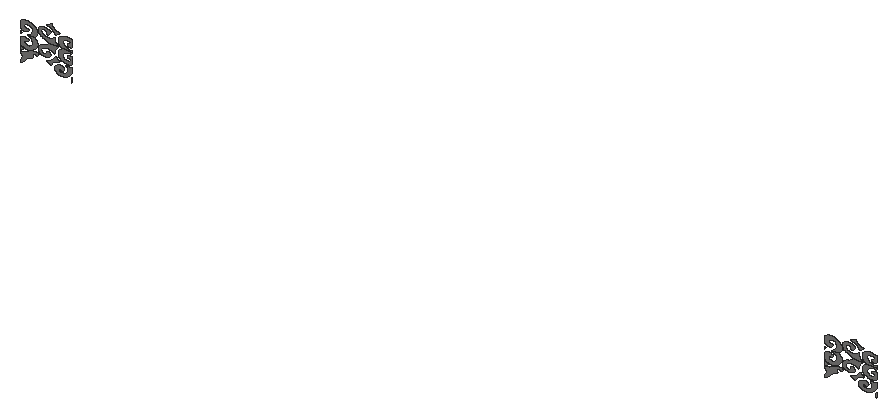
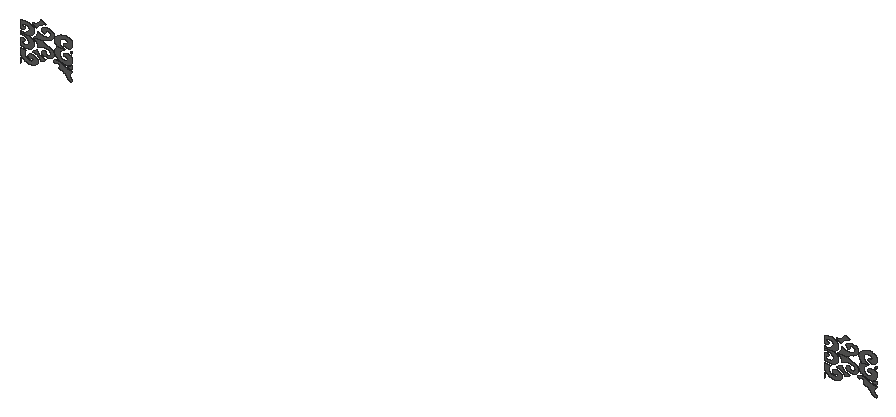
# SketchUp Ruby script. Lengths in inches.
U = 1.inch
M = Sketchup.active_model
def pt(a) = Geom::Point3d.new(a.map { |v| v * U })
def face(e, loops, mat)
  f = e.add_face(loops[0].map { |a| pt(a) })
  loops[1..].each { |l| e.add_face(l.map { |a| pt(a) }).erase! }
  f.material = f.back_material = mat if mat
  f
end
# faces: each face lists its corners as indices into pts; further lists are holes
def faces(e, pts, list, mat = nil) = list.each { |f| face(e, (f[0].is_a?(Array) ? f : [f]).map { |l| l.map { |i| pts[i] } }, mat) }
# xy, xz, yz: faces in a plane at the given z, y or x. An outline is a flat list of corners, or four numbers for a rectangle; further outlines are holes
def ring(l) = l.size == 4 ? [[l[0], l[1]], [l[2], l[1]], [l[2], l[3]], [l[0], l[3]]] : l.each_slice(2).to_a
def flat(e, list, mat, &to3) = list.each { |f| face(e, (f[0].is_a?(Array) ? f : [f]).map { |l| ring(l).map { |u, v| to3.(u, v) } }, mat) }
def xy(e, z, list, mat = nil) = flat(e, list, mat) { |x, y| [x, y, z] }
def xz(e, y, list, mat = nil) = flat(e, list, mat) { |x, z| [x, y, z] }
def yz(e, x, list, mat = nil) = flat(e, list, mat) { |y, z| [x, y, z] }
def lines(e, pts, list) = list.each { |a, b| e.add_line(pt(pts[a]), pt(pts[b])) }
# prism: a flat outline (further loops are holes) pulled along v
def prism(e, loops, v, mat = nil)
  f = face(e, loops, mat); d = Geom::Vector3d.new(v.map { |x| x * U })
  f.pushpull(f.normal.samedirection?(d) ? d.length : -d.length)
end
def box(e, o, s, mat = nil) = prism(e, [[o, [o[0] + s[0], o[1], o[2]], [o[0] + s[0], o[1] + s[1], o[2]], [o[0], o[1] + s[1], o[2]]]], [0, 0, s[2]], mat)
def at(x, y, z, deg = 0) = Geom::Transformation.translation(pt([x, y, z])) * Geom::Transformation.rotation(ORIGIN, Z_AXIS, deg.degrees)
def axes(o, x, y, z) = Geom::Transformation.new([*x, 0, *y, 0, *z, 0, *pt(o).to_a, 1])
def part(name) = M.definitions.add(name)
# library, detail: a bought-in or finely detailed component or shape, given as its bounding box
def library(name, o, s) = part(name).tap { |d| box(d.entities, o, s) }
def detail(e, o, s) = box(e.add_group.entities, o, s)
def put(e, d, t, mat = nil) = e.add_instance(d, t).tap { |i| i.material = mat if mat }
def group(e, t, mat = nil) = e.add_group.tap { |g| g.transformation = t; g.material = mat if mat }.entities
root = M.entities
M.materials.add("[0043_SaddleBrown]4").color = [124, 123, 122]
xz(root,589.17,[[2950.32,580.05,2950.1,580.56,2949.91,581.07,2949.77,581.59,2949.67,582.11,2949.6,582.63,2949.58,583.15,2949.6,583.68,2949.67,584.2,2949.77,584.72,2949.91,585.24,2950.1,585.75,2950.32,586.26],[4200.95,580.05,4200.72,580.56,4200.54,581.07,4200.39,581.59,4200.29,582.11,4200.23,582.63,4200.21,583.15,4200.23,583.68,4200.29,584.2,4200.39,584.72,4200.54,585.24,4200.72,585.75,4200.95,586.26],[2869.93,580.61,2869.93,583.34,2870.95,584.11,2871.81,584.96,2872.49,585.86,2872.98,586.8125,2873.28,587.79,2873.38,588.78,2873.28,589.78,2872.98,590.76,2872.49,591.71,2871.81,592.61,2870.95,593.46,2869.93,594.23,2869.93,595.13,2871.22,595.29,2872.49,595.5,2873.74,595.74,2874.97,596.03,2876.18,596.35,2877.35,596.71,2878.49,597.11,2879.6,597.55,2880.67,598.02,2881.69,598.53,2882.67,599.0625,2883.61,599.63,2884.34,600.07,2885.11,600.47,2885.94,600.83,2886.8,601.16,2887.7,601.46,2888.625,601.71,2889.58,601.92,2890.5625,602.08,2891.56,602.21,2892.57,602.28,2893.58,602.32,2894.6,602.31,2895.41,602.23,2896.17,602.03,2896.85,601.74,2897.4,601.36,2897.79,600.91,2898.01,600.43,2898.05,599.92,2897.9,599.42,2897.57,598.95,2897.08,598.54,2896.46,598.21,2895.73,597.98,2895.62,598.49,2895.3,598.96,2894.79,599.37,2894.125,599.68,2893.35,599.88,2892.52,599.95,2891.7,599.88,2890.92,599.68,2890.26,599.37,2889.75,598.96,2889.43,598.49,2889.32,597.98,2889.28,597.57,2889.25,597.17,2889.24,596.76,2889.25,596.36,2889.28,595.95,2889.32,595.55,2889.39,595.15,2889.47,594.74,2889.5625,594.34,2889.68,593.95,2889.8125,593.55,2889.96,593.15,2888.5,592.79,2887.09,592.36,2885.73,591.86,2884.45,591.3,2883.24,590.67,2882.12,589.99,2881.09,589.26,2880.16,588.48,2879.33,587.65,2878.62,586.79,2878.01,585.89,2877.52,584.97,2877,584.54,2876.45,584.125,2875.89,583.72,2875.3,583.32,2874.69,582.94,2874.06,582.57,2873.42,582.21,2872.76,581.86,2872.07,581.53,2871.375,581.21,2870.66,580.9],[4120.56,580.61,4120.56,583.34,4121.58,584.11,4122.43,584.96,4123.11,585.86,4123.61,586.8125,4123.91,587.79,4124.01,588.78,4123.91,589.78,4123.61,590.76,4123.11,591.71,4122.43,592.61,4121.58,593.46,4120.56,594.23,4120.56,595.13,4121.84,595.29,4123.12,595.5,4124.37,595.74,4125.6,596.03,4126.8,596.35,4127.98,596.71,4129.12,597.11,4130.22,597.55,4131.29,598.02,4132.32,598.53,4133.3,599.0625,4134.23,599.63,4134.96,600.07,4135.74,600.47,4136.56,600.83,4137.42,601.16,4138.32,601.46,4139.25,601.71,4140.21,601.92,4141.1875,602.08,4142.18,602.21,4143.19,602.28,4144.2,602.32,4145.22,602.31,4146.04,602.23,4146.8,602.03,4147.47,601.74,4148.02,601.36,4148.42,600.91,4148.64,600.43,4148.68,599.92,4148.53,599.42,4148.2,598.95,4147.71,598.54,4147.08,598.21,4146.35,597.98,4146.24,598.49,4145.92,598.96,4145.41,599.37,4144.75,599.68,4143.98,599.88,4143.15,599.95,4142.32,599.88,4141.55,599.68,4140.88,599.37,4140.375,598.96,4140.06,598.49,4139.95,597.98,4139.9,597.57,4139.875,597.17,4139.87,596.76,4139.88,596.36,4139.9,595.95,4139.95,595.55,4140.01,595.15,4140.09,594.74,4140.1875,594.34,4140.3,593.95,4140.4375,593.55,4140.59,593.15,4139.125,592.79,4137.71,592.36,4136.36,591.86,4135.08,591.3,4133.87,590.67,4132.75,589.99,4131.72,589.26,4130.79,588.48,4129.96,587.65,4129.24,586.79,4128.64,585.89,4128.15,584.97,4127.625,584.54,4127.08,584.125,4126.51,583.72,4125.92,583.32,4125.32,582.94,4124.69,582.57,4124.04,582.21,4123.38,581.86,4122.7,581.53,4122,581.21,4121.29,580.9],[2933.97,583.36,2932.56,583.46,2931.17,583.66,2929.83,583.96,2927.89,584.61,2926.2,585.48,2924.8125,586.54,2923.78,587.74,2923.15,589.04,2922.93,590.39,2923.15,591.74,2923.78,593.04,2924.8125,594.24,2926.2,595.29,2927.89,596.16,2929.83,596.82,2930.47,597.05,2931.16,597.21,2931.89,597.31,2932.63,597.33,2933.37,597.28,2934.09,597.17,2934.77,596.98,2935.39,596.73,2935.93,596.42,2936.4,596.0625,2936.76,595.66,2937.02,595.23,2937.38,594.85,2937.66,594.45,2937.83,594.02,2937.91,593.58,2937.88,593.14,2937.76,592.7,2937.54,592.28,2937.22,591.89,2936.8125,591.52,2936.33,591.2,2935.77,590.92,2935.16,590.6875,2934.8,590.8,2934.46,590.93,2934.13,591.07,2933.82,591.23,2933.53,591.4,2933.26,591.58,2933.01,591.78,2932.79,591.98,2932.58,592.19,2932.4,592.41,2932.25,592.64,2932.12,592.87,2931.35,592.59,2930.6875,592.22,2930.14,591.79,2929.74,591.3,2929.49,590.77,2929.41,590.23,2929.49,589.68,2929.74,589.15,2930.14,588.66,2930.6875,588.23,2931.35,587.86,2932.12,587.58,2933.05,587.56,2933.98,587.58,2934.91,587.64,2935.83,587.75,2936.73,587.9,2937.61,588.09,2938.47,588.32,2939.29,588.58,2940.09,588.89,2940.84,589.23,2941.55,589.6,2942.21,590,2942.79,590.79,2943.26,591.6,2943.61,592.43,2943.83,593.28,2943.93,594.14,2943.9,595,2943.75,595.85,2943.47,596.7,2943.07,597.52,2942.55,598.32,2941.92,599.09,2941.17,599.82,2941.93,599.65,2942.72,599.53,2943.51,599.46,2944.32,599.42,2945.12,599.43,2945.92,599.48,2946.72,599.57,2947.49,599.7,2948.25,599.88,2948.97,600.09,2949.67,600.35,2950.32,600.64,2950.32,593.03,2949.96,592.48,2949.58,591.93,2949.18,591.39,2948.77,590.85,2948.35,590.3125,2947.9,589.78,2947.45,589.26,2946.97,588.74,2946.49,588.23,2945.99,587.72,2945.47,587.21,2944.94,586.71,2944.08,586.02,2943.1,585.38,2942,584.82,2940.8125,584.34,2939.54,583.95,2938.2,583.66,2936.81,583.46,2935.39,583.36],
  [4184.6,583.36,4183.18,583.46,4181.79,583.66,4180.45,583.96,4178.52,584.61,4176.83,585.48,4175.4375,586.54,4174.41,587.74,4173.77,589.04,4173.56,590.39,4173.77,591.74,4174.41,593.04,4175.4375,594.24,4176.83,595.29,4178.52,596.16,4180.45,596.82,4181.1,597.05,4181.79,597.21,4182.51,597.31,4183.26,597.33,4184,597.28,4184.71,597.17,4185.39,596.98,4186.01,596.73,4186.56,596.42,4187.02,596.0625,4187.39,595.66,4187.64,595.23,4188.01,594.85,4188.28,594.45,4188.46,594.02,4188.53,593.58,4188.51,593.14,4188.38,592.7,4188.16,592.28,4187.84,591.89,4187.4375,591.52,4186.95,591.2,4186.4,590.92,4185.78,590.6875,4185.43,590.8,4185.09,590.93,4184.76,591.07,4184.45,591.23,4184.16,591.4,4183.89,591.58,4183.64,591.78,4183.41,591.98,4183.21,592.19,4183.03,592.41,4182.87,592.64,4182.74,592.87,4181.98,592.59,4181.3125,592.22,4180.77,591.79,4180.36,591.3,4180.12,590.77,4180.03,590.23,4180.12,589.68,4180.36,589.15,4180.77,588.66,4181.3125,588.23,4181.98,587.86,4182.74,587.58,4183.68,587.56,4184.61,587.58,4185.54,587.64,4186.45,587.75,4187.36,587.9,4188.24,588.09,4189.09,588.32,4189.92,588.58,4190.71,588.89,4191.46,589.23,4192.17,589.6,4192.83,590,4193.42,590.79,4193.89,591.6,4194.23,592.43,4194.46,593.28,4194.56,594.14,4194.53,595,4194.375,595.85,4194.1,596.7,4193.69,597.52,4193.17,598.32,4192.54,599.09,4191.8,599.82,4192.56,599.65,4193.34,599.53,4194.14,599.46,4194.94,599.42,4195.75,599.43,4196.55,599.48,4197.34,599.57,4198.12,599.7,4198.87,599.88,4199.6,600.09,4200.29,600.35,4200.95,600.64,4200.95,593.03,4200.58,592.48,4200.2,591.93,4199.81,591.39,4199.4,590.85,4198.97,590.3125,4198.53,589.78,4198.07,589.26,4197.6,588.74,4197.11,588.23,4196.61,587.72,4196.1,587.21,4195.57,586.71,4194.71,586.02,4193.73,585.38,4192.63,584.82,4191.4375,584.34,4190.16,583.95,4188.82,583.66,4187.43,583.46,4186.02,583.36],[2918.45,593.19,2917.9,593.51,2917.34,593.83,2916.78,594.14,2916.2,594.45,2915.61,594.75,2915.02,595.04,2914.42,595.32,2913.81,595.6,2913.1875,595.875,2912.5625,596.14,2911.93,596.4,2911.29,596.65,2912.89,597.11,2914.43,597.64,2915.9,598.25,2917.28,598.92,2918.57,599.66,2919.77,600.46,2920.86,601.32,2921.83,602.23,2922.6875,603.18,2923.42,604.17,2924.02,605.1875,2924.49,606.23,2925.02,605.83,2925.5625,605.43,2926.11,605.04,2926.67,604.66,2927.83,603.9,2928.42,603.53,2929.02,603.17,2929.63,602.8125,2930.25,602.46,2930.88,602.12,2931.52,601.78,2929.85,601.54,2928.24,601.2,2926.69,600.75,2925.23,600.2,2923.88,599.56,2922.64,598.83,2921.55,598.02,2920.59,597.15,2919.8,596.22,2919.17,595.24,2918.72,594.23],[4169.08,593.19,4168.53,593.51,4167.97,593.83,4167.4,594.14,4166.82,594.45,4166.24,594.75,4165.65,595.04,4164.43,595.6,4163.8125,595.875,4163.1875,596.14,4162.55,596.4,4161.91,596.65,4163.51,597.11,4165.05,597.64,4166.52,598.25,4167.91,598.92,4169.2,599.66,4170.39,600.46,4171.48,601.32,4172.46,602.23,4173.3125,603.18,4174.04,604.17,4174.65,605.1875,4175.12,606.23,4175.65,605.83,4176.1875,605.43,4176.74,605.04,4177.3,604.66,4177.87,604.28,4178.45,603.9,4179.04,603.53,4179.65,603.17,4180.26,602.8125,4180.875,602.46,4181.5,602.12,4182.14,601.78,4180.48,601.54,4178.86,601.2,4177.32,600.75,4175.86,600.2,4174.5,599.56,4173.27,598.83,4172.17,598.02,4171.22,597.15,4170.43,596.22,4169.8,595.24,4169.35,594.23],[2869.93,598.4,2869.93,602.86,2870.29,602.55,2870.68,602.26,2871.09,601.99,2871.54,601.73,2872.02,601.49,2872.52,601.28,2873.04,601.08,2873.59,600.91,2874.15,600.76,2874.73,600.64,2875.32,600.54,2875.92,600.46,2875.55,600.18,2875.15,599.91,2874.72,599.66,2874.27,599.43,2873.79,599.22,2873.28,599.03,2872.76,598.87,2872.22,598.73,2871.66,598.61,2871.1,598.51,2870.52,598.45],[4120.56,598.4,4120.56,602.86,4120.91,602.55,4121.3,602.26,4121.72,601.99,4122.17,601.73,4122.64,601.49,4123.15,601.28,4123.67,601.08,4124.21,600.91,4124.77,600.76,4125.35,600.64,4125.94,600.54,4126.54,600.46,4126.17,600.18,4125.78,599.91,4125.35,599.66,4124.89,599.43,4124.41,599.22,4123.91,599.03,4123.39,598.87,4122.85,598.73,4122.29,598.61,4121.72,598.51,4121.14,598.45],
  [2907.9,601.54,2905.91,601.66,2904,602.02,2902.25,602.62,2900.73,603.42,2899.5,604.39,2898.63,605.5,2898.14,606.69,2897.99,607.57,2897.97,608.46,2898.07,609.34,2898.3,610.21,2898.65,611.07,2899.13,611.9,2899.72,612.71,2900.42,613.48,2901.23,614.21,2902.14,614.9,2903.15,615.53,2904.24,616.11,2905.39,616.38,2906.52,616.6875,2907.61,617.04,2908.67,617.42,2909.7,617.84,2910.6875,618.3,2911.63,618.79,2912.53,619.31,2913.375,619.86,2914.17,620.4375,2914.91,621.04,2915.6,621.67,2929.37,621.67,2928.39,620.92,2927.48,620.13,2926.66,619.3,2925.92,618.45,2925.27,617.57,2924.7,616.67,2924.23,615.75,2923.85,614.8125,2923.57,613.86,2923.38,612.9,2923.29,611.9375,2923.3,610.97,2922.72,611.43,2922.08,611.87,2921.4,612.28,2920.68,612.66,2919.91,613,2919.1,613.3125,2918.26,613.59,2917.39,613.83,2916.5,614.03,2915.58,614.1875,2914.65,614.31,2913.71,614.39,2912.08,614.41,2910.47,614.28,2908.91,613.99,2907.45,613.55,2906.12,612.98,2904.94,612.29,2903.96,611.49,2903.2,610.61,2902.67,609.66,2902.39,608.68,2902.37,607.68,2902.6,606.69,2902.85,606.21,2903.25,605.76,2903.77,605.36,2904.4,605.02,2905.11,604.76,2905.89,604.59,2906.71,604.5,2907.54,604.51,2908.36,604.61,2909.13,604.8,2909.84,605.07,2910.45,605.41,2910.61,605.62,2910.76,605.83,2910.88,606.05,2910.98,606.27,2911.07,606.5,2911.13,606.73,2911.17,606.96,2911.19,607.1875,2911.2,607.42,2911.18,607.65,2911.14,607.88,2911.08,608.11,2911.04,608.32,2911.07,608.53,2911.15,608.74,2911.29,608.93,2911.48,609.11,2911.72,609.26,2912,609.39,2912.31,609.48,2912.64,609.54,2912.98,609.56,2913.33,609.55,2913.67,609.5,2914.27,609.21,2914.82,608.88,2915.3125,608.51,2915.73,608.11,2916.08,607.69,2916.35,607.25,2916.54,606.79,2916.65,606.32,2916.67,605.84,2916.61,605.37,2916.47,604.91,2916.25,604.45,2915.04,603.47,2913.54,602.66,2911.8,602.05,2909.89,601.67],[4158.53,601.54,4156.53,601.66,4154.62,602.02,4152.87,602.62,4151.35,603.42,4150.13,604.39,4149.25,605.5,4148.76,606.69,4148.61,607.57,4148.59,608.46,4148.7,609.34,4148.93,610.21,4149.28,611.07,4149.75,611.9,4150.34,612.71,4151.05,613.48,4151.86,614.21,4152.77,614.9,4153.77,615.53,4154.86,616.11,4156.02,616.38,4157.14,616.6875,4158.24,617.04,4159.3,617.42,4160.33,617.84,4161.3125,618.3,4162.25,618.79,4163.15,619.31,4164,619.86,4164.8,620.4375,4165.54,621.04,4166.22,621.67,4179.99,621.67,4179.01,620.92,4178.11,620.13,4177.28,619.3,4176.54,618.45,4175.89,617.57,4175.33,616.67,4174.86,615.75,4174.48,614.8125,4174.2,613.86,4174.01,612.9,4173.92,611.9375,4173.92,610.97,4173.34,611.43,4172.71,611.87,4172.03,612.28,4171.3,612.66,4170.53,613,4169.73,613.3125,4168.89,613.59,4168.02,613.83,4167.125,614.03,4166.21,614.1875,4165.28,614.31,4164.33,614.39,4162.71,614.41,4161.1,614.28,4159.54,613.99,4158.08,613.55,4156.74,612.98,4155.57,612.29,4154.59,611.49,4153.83,610.61,4153.3,609.66,4153.02,608.68,4152.99,607.68,4153.22,606.69,4153.48,606.21,4153.87,605.76,4154.39,605.36,4155.02,605.02,4155.74,604.76,4156.52,604.59,4157.34,604.5,4158.17,604.51,4158.98,604.61,4159.76,604.8,4160.46,605.07,4161.08,605.41,4161.24,605.62,4161.38,605.83,4161.5,606.05,4161.61,606.27,4161.69,606.5,4161.75,606.73,4161.8,606.96,4161.82,607.1875,4161.82,607.42,4161.8,607.65,4161.76,607.88,4161.7,608.11,4161.67,608.32,4161.69,608.53,4161.77,608.74,4161.91,608.93,4162.11,609.11,4162.35,609.26,4162.625,609.39,4162.93,609.48,4163.27,609.54,4163.61,609.56,4163.95,609.55,4164.29,609.5,4164.9,609.21,4165.45,608.88,4165.9375,608.51,4166.36,608.11,4166.7,607.69,4166.97,607.25,4167.16,606.79,4167.27,606.32,4167.3,605.84,4167.24,605.37,4167.09,604.91,4166.87,604.45,4165.67,603.47,4164.16,602.66,4162.42,602.05,4160.52,601.67],[2880.76,601.96,2879.19,601.97,2877.65,602.14,2876.16,602.44,2874.77,602.89,2873.5,603.45,2872.38,604.13,2871.45,604.91,2870.72,605.76,2870.21,606.67,2869.93,607.62,2869.93,614.39,2870.39,615.13,2871.07,615.8,2871.95,616.38,2872.98,616.85,2874.14,617.19,2875.38,617.38,2876.67,617.44,2877.94,617.34,2879.16,617.09,2880.29,616.71,2881.28,616.21,2882.09,615.6,2882.33,615.33,2882.49,615.03,2882.56,614.73,2882.54,614.42,2882.43,614.11,2882.23,613.83,2881.95,613.57,2881.59,613.35,2881.18,613.17,2880.73,613.04,2880.24,612.96,2879.74,612.9375,2879.07,612.91,2878.42,612.8125,2877.8125,612.65,2877.26,612.42,2876.78,612.14,2876.38,611.81,2876.08,611.44,2875.89,611.05,2875.81,610.64,2875.85,610.23,2876.01,609.83,2876.27,609.45,2876.65,608.8,2877.22,608.21,2877.97,607.6875,2878.86,607.26,2879.87,606.95,2880.95,606.75,2882.07,606.69,2883.2,606.76,2884.28,606.95,2885.28,607.27,2886.7,608.37,2887.84,609.6,2888.65,610.92,2889.12,612.3,2889.25,613.7,2889.02,615.1,2888.45,616.47,2887.54,617.76,2886.32,618.96,2884.82,620.02,2883.07,620.9375,2881.12,621.67,2892.0625,621.67,2893.89,620.09,2895.29,618.34,2896.22,616.49,2896.66,614.57,2896.6,612.625,2896.04,610.71,2895,608.88,2893.5,607.17,2891.58,605.625,2889.29,604.29,2886.68,603.1875,2883.82,602.36,2882.32,602.08],[4131.39,601.96,4129.82,601.97,4128.27,602.14,4126.79,602.44,4125.39,602.89,4124.12,603.45,4123.01,604.13,4122.08,604.91,4121.35,605.76,4120.84,606.67,4120.56,607.62,4120.56,614.39,4121.02,615.13,4121.7,615.8,4122.57,616.38,4123.61,616.85,4124.77,617.19,4126.01,617.38,4127.29,617.44,4128.57,617.34,4129.79,617.09,4130.91,616.71,4131.9,616.21,4132.72,615.6,4132.96,615.33,4133.12,615.03,4133.18,614.73,4133.16,614.42,4133.05,614.11,4132.85,613.83,4132.57,613.57,4132.22,613.35,4131.81,613.17,4131.35,613.04,4130.86,612.96,4130.36,612.9375,4129.7,612.91,4129.05,612.8125,4128.4375,612.65,4127.88,612.42,4127.4,612.14,4127,611.81,4126.71,611.44,4126.52,611.05,4126.44,610.64,4126.48,610.23,4126.63,609.83,4126.89,609.45,4127.27,608.8,4127.85,608.21,4128.59,607.6875,4129.48,607.26,4130.49,606.95,4131.57,606.75,4132.7,606.69,4133.82,606.76,4134.9,606.95,4135.91,607.27,4137.33,608.37,4138.46,609.6,4139.27,610.92,4139.75,612.3,4139.87,613.7,4139.64,615.1,4139.07,616.47,4138.17,617.76,4136.95,618.96,4135.45,620.02,4133.7,620.9375,4131.74,621.67,4142.6875,621.67,4144.52,620.09,4145.91,618.34,4146.84,616.49,4147.28,614.57,4147.23,612.625,4146.67,610.71,4145.63,608.88,4144.13,607.17,4142.21,605.625,4139.91,604.29,4137.31,603.1875,4134.45,602.36,4132.94,602.08],[2942.6,603.16,2939.9,603.34,2937.31,603.85,2934.93,604.66,2932.86,605.74,2931.17,607.05,2929.94,608.54,2929.21,610.15,2929.02,611.82,2929.35,613.47,2929.43,614.32,2929.64,615.16,2929.97,615.98,2930.42,616.78,2930.98,617.56,2931.66,618.3,2932.45,618.99,2933.34,619.64,2934.32,620.24,2935.38,620.78,2936.52,621.26,2937.73,621.67,2950.32,621.67,2950.32,619.15,2950.02,619.38,2949.68,619.6,2949.3,619.78,2948.88,619.9375,2948.4375,620.0625,2947.98,620.15,2947.5,620.21,2947.01,620.23,2946.53,620.22,2946.05,620.17,2945.58,620.09,2945.13,619.97,2944.05,619.61,2943.02,619.2,2942.03,618.75,2941.1,618.26,2940.24,617.73,2939.43,617.15,2938.7,616.55,2938.04,615.91,2937.45,615.25,2936.95,614.5625,2936.52,613.85,2936.1875,613.13,2935.99,612.42,2935.96,611.71,2936.1,610.99,2936.4,610.3,2936.87,609.64,2937.48,609.04,2938.24,608.49,2939.11,608.01,2940.09,607.62,2941.15,607.32,2942.27,607.11,2943.42,607.01,2944.49,607.04,2945.5,607.24,2946.41,607.58,2947.16,608.04,2947.7,608.61,2948,609.23,2948.04,609.89,2947.82,610.53,2947.35,611.12,2946.66,611.62,2945.8,612,2944.8,612.24,2944.56,612.22,2944.3125,612.24,2944.07,612.27,2943.85,612.34,2943.65,612.42,2943.47,612.53,2943.33,612.65,2943.22,612.79,2943.15,612.93,2943.125,613.08,2943.14,613.24,2943.2,613.38,2943.48,613.79,2943.875,614.17,2944.36,614.5,2944.92,614.78,2945.56,615,2946.24,615.15,2946.95,615.23,2947.68,615.24,2948.4,615.18,2949.09,615.05,2949.74,614.85,2950.32,614.58,2950.32,604.55,2947.92,603.77,2945.31,603.3],
  [4193.22,603.16,4190.52,603.34,4187.93,603.85,4185.55,604.66,4183.48,605.74,4181.8,607.05,4180.57,608.54,4179.84,610.15,4179.64,611.82,4179.98,613.47,4180.06,614.32,4180.26,615.16,4180.59,615.98,4181.04,616.78,4181.61,617.56,4182.29,618.3,4183.08,618.99,4183.96,619.64,4184.94,620.24,4186.01,620.78,4187.15,621.26,4188.36,621.67,4200.95,621.67,4200.95,619.15,4200.65,619.38,4200.3,619.6,4199.92,619.78,4199.51,619.9375,4199.0625,620.0625,4198.6,620.15,4198.125,620.21,4197.64,620.23,4197.15,620.22,4196.67,620.17,4196.2,620.09,4195.76,619.97,4194.68,619.61,4193.64,619.2,4192.66,618.75,4191.73,618.26,4190.86,617.73,4190.06,617.15,4189.32,616.55,4188.66,615.91,4188.08,615.25,4187.57,614.5625,4187.15,613.85,4186.8125,613.13,4186.61,612.42,4186.58,611.71,4186.72,610.99,4187.03,610.3,4187.49,609.64,4188.11,609.04,4188.86,608.49,4189.74,608.01,4190.71,607.62,4191.77,607.32,4192.89,607.11,4194.05,607.01,4195.11,607.04,4196.13,607.24,4197.04,607.58,4197.79,608.04,4198.33,608.61,4198.625,609.23,4198.67,609.89,4198.45,610.53,4197.98,611.12,4197.29,611.62,4196.42,612,4195.43,612.24,4195.18,612.22,4194.9375,612.24,4194.7,612.27,4194.47,612.34,4194.27,612.42,4194.1,612.53,4193.95,612.65,4193.84,612.79,4193.78,612.93,4193.75,613.08,4193.77,613.24,4193.82,613.38,4194.11,613.79,4194.5,614.17,4194.98,614.5,4195.55,614.78,4196.18,615,4196.86,615.15,4197.58,615.23,4198.3,615.24,4199.02,615.18,4199.71,615.05,4200.36,614.85,4200.95,614.58,4200.95,604.55,4198.54,603.77,4195.93,603.3],[2869.93,620.2,2869.93,621.67,2872.33,621.67,2872.02,621.66,2871.71,621.62,2871.41,621.5625,2871.13,621.48,2870.87,621.37,2870.63,621.24,2870.43,621.1,2870.25,620.9375,2870.12,620.76,2870.01,620.58,2869.95,620.39],[4120.56,620.2,4120.56,621.67,4122.96,621.67,4122.64,621.66,4122.33,621.62,4122.04,621.5625,4121.76,621.48,4121.5,621.37,4121.26,621.24,4121.05,621.1,4120.88,620.9375,4120.74,620.76,4120.64,620.58,4120.58,620.39],[2869.93,621.67,2872.33,621.67,2872.02,621.6875,2871.71,621.72,2871.41,621.79,2871.13,621.87,2870.87,621.98,2870.63,622.1,2870.43,622.25,2870.25,622.41,2870.12,622.58,2870.01,622.76,2869.95,622.95,2869.93,623.15],[2881.12,621.67,2892.0625,621.67,2893.89,623.26,2895.29,625,2896.22,626.86,2896.66,628.78,2896.6,630.72,2896.04,632.63,2895,634.47,2893.5,636.18,2891.58,637.72,2889.29,639.06,2886.68,640.16,2883.82,640.99,2882.32,641.26,2880.76,641.39,2879.19,641.37,2877.65,641.21,2876.16,640.9,2874.77,640.46,2873.5,639.89,2872.38,639.21,2871.45,638.4375,2870.72,637.59,2870.21,636.67,2869.93,635.73,2869.93,628.95,2870.39,628.22,2871.07,627.55,2871.95,626.97,2872.98,626.5,2874.14,626.16,2875.38,625.96,2876.67,625.91,2877.94,626.01,2879.16,626.25,2880.29,626.63,2881.28,627.14,2882.09,627.75,2882.33,628.02,2882.49,628.3125,2882.56,628.62,2882.54,628.93,2882.43,629.23,2882.23,629.52,2881.95,629.77,2881.59,630,2881.18,630.17,2880.73,630.31,2880.24,630.38,2879.74,630.41,2879.07,630.44,2878.42,630.53,2877.8125,630.7,2877.26,630.93,2876.78,631.21,2876.38,631.54,2876.08,631.91,2875.89,632.3,2875.81,632.71,2875.85,633.12,2876.01,633.51,2876.27,633.89,2876.65,634.54,2877.22,635.14,2877.97,635.66,2878.86,636.08,2879.87,636.4,2880.95,636.59,2882.07,636.66,2883.2,636.59,2884.28,636.4,2885.28,636.08,2886.7,634.97,2887.84,633.75,2888.65,632.43,2889.12,631.05,2889.25,629.64,2889.02,628.24,2888.45,626.875,2887.54,625.58,2886.32,624.39,2884.82,623.32,2883.07,622.41],
  [2915.6,621.67,2929.37,621.67,2928.39,622.43,2927.48,623.22,2926.66,624.04,2925.92,624.89,2925.27,625.77,2924.7,626.68,2924.23,627.6,2923.85,628.53,2923.57,629.48,2923.38,630.44,2923.29,631.41,2923.3,632.375,2922.72,631.91,2922.08,631.47,2921.4,631.07,2920.68,630.6875,2919.91,630.34,2919.1,630.03,2918.26,629.76,2917.39,629.52,2916.5,629.32,2915.58,629.16,2914.65,629.04,2913.71,628.96,2912.08,628.9375,2910.47,629.07,2908.91,629.36,2907.45,629.79,2906.12,630.37,2904.94,631.06,2903.96,631.86,2903.2,632.74,2902.67,633.68,2902.39,634.67,2902.37,635.67,2902.6,636.65,2902.85,637.14,2903.25,637.59,2903.77,637.99,2904.4,638.32,2905.11,638.58,2905.89,638.76,2906.71,638.84,2907.54,638.84,2908.36,638.74,2909.13,638.55,2909.84,638.28,2910.45,637.9375,2910.61,637.73,2910.76,637.51,2910.88,637.29,2910.98,637.07,2911.07,636.85,2911.13,636.62,2911.17,636.39,2911.19,636.16,2911.2,635.93,2911.18,635.7,2911.14,635.47,2911.08,635.24,2911.04,635.03,2911.07,634.82,2911.15,634.61,2911.29,634.42,2911.48,634.24,2911.72,634.09,2912,633.96,2912.31,633.87,2912.64,633.81,2912.98,633.78,2913.33,633.79,2913.67,633.84,2914.27,634.14,2914.82,634.47,2915.3125,634.84,2915.73,635.23,2916.08,635.66,2916.35,636.1,2916.54,636.56,2916.65,637.03,2916.67,637.5,2916.61,637.97,2916.47,638.44,2916.25,638.89,2915.04,639.875,2913.54,640.6875,2911.8,641.29,2909.89,641.67,2907.9,641.8,2905.91,641.6875,2904,641.32,2902.25,640.73,2900.73,639.93,2899.5,638.95,2898.63,637.85,2898.14,636.65,2897.99,635.77,2897.97,634.89,2898.07,634.01,2898.3,633.14,2898.65,632.28,2899.13,631.44,2899.72,630.64,2900.42,629.86,2901.23,629.13,2902.14,628.45,2903.15,627.81,2904.24,627.24,2905.39,626.97,2906.52,626.66,2907.61,626.31,2908.67,625.92,2909.7,625.5,2910.6875,625.05,2911.63,624.56,2912.53,624.04,2913.375,623.49,2914.17,622.91,2914.91,622.3],[2937.73,621.67,2950.32,621.67,2950.32,624.2,2950.02,623.96,2949.68,623.75,2949.3,623.56,2948.88,623.41,2948.4375,623.28,2947.98,623.19,2947.5,623.14,2947.01,623.11,2946.53,623.125,2946.05,623.18,2945.58,623.26,2945.13,623.375,2944.05,623.74,2943.02,624.14,2942.03,624.59,2941.1,625.09,2940.24,625.62,2939.43,626.19,2938.7,626.8,2938.04,627.43,2937.45,628.1,2936.95,628.78,2936.52,629.49,2936.1875,630.22,2935.99,630.92,2935.96,631.64,2936.1,632.35,2936.4,633.04,2936.87,633.7,2937.48,634.3125,2938.24,634.86,2939.11,635.33,2940.09,635.73,2941.15,636.03,2942.27,636.23,2943.42,636.34,2944.49,636.3,2945.5,636.11,2946.41,635.77,2947.16,635.3,2947.7,634.74,2948,634.11,2948.04,633.46,2947.82,632.82,2947.35,632.23,2946.66,631.73,2945.8,631.35,2944.8,631.11,2944.56,631.125,2944.3125,631.11,2944.07,631.07,2943.85,631.01,2943.65,630.92,2943.47,630.82,2943.33,630.69,2943.22,630.56,2943.15,630.41,2943.125,630.26,2943.14,630.11,2943.2,629.96,2943.48,629.55,2943.875,629.18,2944.36,628.85,2944.92,628.57,2945.56,628.35,2946.24,628.2,2946.95,628.11,2947.68,628.1,2948.4,628.16,2949.09,628.3,2949.74,628.5,2950.32,628.76,2950.32,638.8,2947.92,639.57,2945.31,640.04,2942.6,640.1875,2939.9,640,2937.31,639.5,2934.93,638.6875,2932.86,637.61,2931.17,636.29,2929.94,634.8,2929.21,633.2,2929.02,631.53,2929.35,629.875,2929.43,629.03,2929.64,628.1875,2929.97,627.36,2930.42,626.5625,2930.98,625.79,2931.66,625.05,2932.45,624.35,2933.34,623.7,2934.32,623.1,2935.38,622.5625,2936.52,622.09],[4120.56,621.67,4122.96,621.67,4122.64,621.6875,4122.33,621.72,4122.04,621.79,4121.76,621.87,4121.5,621.98,4121.26,622.1,4121.05,622.25,4120.88,622.41,4120.74,622.58,4120.64,622.76,4120.58,622.95,4120.56,623.15],[4131.74,621.67,4142.6875,621.67,4144.52,623.26,4145.91,625,4146.84,626.86,4147.28,628.78,4147.23,630.72,4146.67,632.63,4145.63,634.47,4144.13,636.18,4142.21,637.72,4139.91,639.06,4137.31,640.16,4134.45,640.99,4132.94,641.26,4131.39,641.39,4129.82,641.37,4128.27,641.21,4126.79,640.9,4125.39,640.46,4124.12,639.89,4123.01,639.21,4122.08,638.4375,4121.35,637.59,4120.84,636.67,4120.56,635.73,4120.56,628.95,4121.02,628.22,4121.7,627.55,4122.57,626.97,4123.61,626.5,4124.77,626.16,4126.01,625.96,4127.29,625.91,4128.57,626.01,4129.79,626.25,4130.91,626.63,4131.9,627.14,4132.72,627.75,4132.96,628.02,4133.12,628.3125,4133.18,628.62,4133.16,628.93,4133.05,629.23,4132.85,629.52,4132.57,629.77,4132.22,630,4131.81,630.17,4131.35,630.31,4130.86,630.38,4130.36,630.41,4129.7,630.44,4129.05,630.53,4128.4375,630.7,4127.88,630.93,4127.4,631.21,4127,631.54,4126.71,631.91,4126.52,632.3,4126.44,632.71,4126.48,633.12,4126.63,633.51,4126.89,633.89,4127.27,634.54,4127.85,635.14,4128.59,635.66,4129.48,636.08,4130.49,636.4,4131.57,636.59,4132.7,636.66,4133.82,636.59,4134.9,636.4,4135.91,636.08,4137.33,634.97,4138.46,633.75,4139.27,632.43,4139.75,631.05,4139.87,629.64,4139.64,628.24,4139.07,626.875,4138.17,625.58,4136.95,624.39,4135.45,623.32,4133.7,622.41],[4166.22,621.67,4179.99,621.67,4179.01,622.43,4178.11,623.22,4177.28,624.04,4176.54,624.89,4175.89,625.77,4175.33,626.68,4174.86,627.6,4174.48,628.53,4174.2,629.48,4174.01,630.44,4173.92,631.41,4173.92,632.375,4173.34,631.91,4172.71,631.47,4172.03,631.07,4171.3,630.6875,4170.53,630.34,4169.73,630.03,4168.89,629.76,4168.02,629.52,4167.125,629.32,4166.21,629.16,4165.28,629.04,4164.33,628.96,4162.71,628.9375,4161.1,629.07,4159.54,629.36,4158.08,629.79,4156.74,630.37,4155.57,631.06,4154.59,631.86,4153.83,632.74,4153.3,633.68,4153.02,634.67,4152.99,635.67,4153.22,636.65,4153.48,637.14,4153.87,637.59,4154.39,637.99,4155.02,638.32,4155.74,638.58,4156.52,638.76,4157.34,638.84,4158.17,638.84,4158.98,638.74,4159.76,638.55,4160.46,638.28,4161.08,637.9375,4161.24,637.73,4161.38,637.51,4161.5,637.29,4161.61,637.07,4161.69,636.85,4161.75,636.62,4161.8,636.39,4161.82,636.16,4161.82,635.93,4161.8,635.7,4161.76,635.47,4161.7,635.24,4161.67,635.03,4161.69,634.82,4161.77,634.61,4161.91,634.42,4162.11,634.24,4162.35,634.09,4162.625,633.96,4162.93,633.87,4163.27,633.81,4163.61,633.78,4163.95,633.79,4164.29,633.84,4164.9,634.14,4165.45,634.47,4165.9375,634.84,4166.36,635.23,4166.7,635.66,4166.97,636.1,4167.16,636.56,4167.27,637.03,4167.3,637.5,4167.24,637.97,4167.09,638.44,4166.87,638.89,4165.67,639.875,4164.16,640.6875,4162.42,641.29,4160.52,641.67,4158.53,641.8,4156.53,641.6875,4154.62,641.32,4152.87,640.73,4151.35,639.93,4150.13,638.95,4149.25,637.85,4148.76,636.65,4148.61,635.77,4148.59,634.89,4148.7,634.01,4148.93,633.14,4149.28,632.28,4149.75,631.44,4150.34,630.64,4151.05,629.86,4151.86,629.13,4152.77,628.45,4153.77,627.81,4154.86,627.24,4156.02,626.97,4157.14,626.66,4158.24,626.31,4159.3,625.92,4160.33,625.5,4161.3125,625.05,4162.25,624.56,4163.15,624.04,4164,623.49,4164.8,622.91,4165.54,622.3],
  [4188.36,621.67,4200.95,621.67,4200.95,624.2,4200.65,623.96,4200.3,623.75,4199.92,623.56,4199.51,623.41,4199.0625,623.28,4198.6,623.19,4198.125,623.14,4197.64,623.11,4197.15,623.125,4196.67,623.18,4196.2,623.26,4195.76,623.375,4194.68,623.74,4193.64,624.14,4192.66,624.59,4191.73,625.09,4190.86,625.62,4190.06,626.19,4189.32,626.8,4188.66,627.43,4188.08,628.1,4187.57,628.78,4187.15,629.49,4186.8125,630.22,4186.61,630.92,4186.58,631.64,4186.72,632.35,4187.03,633.04,4187.49,633.7,4188.11,634.3125,4188.86,634.86,4189.74,635.33,4190.71,635.73,4191.77,636.03,4192.89,636.23,4194.05,636.34,4195.11,636.3,4196.13,636.11,4197.04,635.77,4197.79,635.3,4198.33,634.74,4198.625,634.11,4198.67,633.46,4198.45,632.82,4197.98,632.23,4197.29,631.73,4196.42,631.35,4195.43,631.11,4195.18,631.125,4194.9375,631.11,4194.7,631.07,4194.47,631.01,4194.27,630.92,4194.1,630.82,4193.95,630.69,4193.84,630.56,4193.78,630.41,4193.75,630.26,4193.77,630.11,4193.82,629.96,4194.11,629.55,4194.5,629.18,4194.98,628.85,4195.55,628.57,4196.18,628.35,4196.86,628.2,4197.58,628.11,4198.3,628.1,4199.02,628.16,4199.71,628.3,4200.36,628.5,4200.95,628.76,4200.95,638.8,4198.54,639.57,4195.93,640.04,4193.22,640.1875,4190.52,640,4187.93,639.5,4185.55,638.6875,4183.48,637.61,4181.8,636.29,4180.57,634.8,4179.84,633.2,4179.64,631.53,4179.98,629.875,4180.06,629.03,4180.26,628.1875,4180.59,627.36,4181.04,626.5625,4181.61,625.79,4182.29,625.05,4183.08,624.35,4183.96,623.7,4184.94,623.1,4186.01,622.5625,4187.15,622.09],[2924.49,637.11,2925.02,637.51,2925.5625,637.91,2926.11,638.3,2926.67,638.6875,2927.25,639.07,2927.83,639.44,2928.42,639.8125,2929.02,640.18,2929.63,640.53,2930.25,640.88,2930.88,641.23,2931.52,641.57,2929.85,641.8,2928.24,642.15,2926.69,642.6,2925.23,643.15,2923.88,643.79,2922.64,644.52,2921.55,645.32,2920.59,646.2,2919.8,647.125,2919.17,648.1,2918.72,649.12,2918.45,650.15,2917.9,649.83,2917.34,649.51,2916.78,649.2,2916.2,648.9,2915.61,648.6,2915.02,648.31,2914.42,648.02,2913.81,647.74,2913.1875,647.47,2912.5625,647.21,2911.93,646.95,2911.29,646.7,2912.89,646.24,2914.43,645.7,2915.9,645.1,2917.28,644.42,2918.57,643.68,2919.77,642.88,2920.86,642.03,2921.83,641.12,2922.6875,640.17,2923.42,639.18,2924.02,638.16],[4175.12,637.11,4175.65,637.51,4176.1875,637.91,4176.74,638.3,4177.3,638.6875,4177.87,639.07,4178.45,639.44,4179.04,639.8125,4179.65,640.18,4180.26,640.53,4180.875,640.88,4181.5,641.23,4182.14,641.57,4180.48,641.8,4178.86,642.15,4177.32,642.6,4175.86,643.15,4174.5,643.79,4173.27,644.52,4172.17,645.32,4171.22,646.2,4170.43,647.125,4169.8,648.1,4169.35,649.12,4169.08,650.15,4168.53,649.83,4167.97,649.51,4167.4,649.2,4166.24,648.6,4165.65,648.31,4165.04,648.02,4164.43,647.74,4163.8125,647.47,4163.1875,647.21,4162.55,646.95,4161.91,646.7,4163.51,646.24,4165.05,645.7,4166.52,645.1,4167.91,644.42,4169.2,643.68,4170.39,642.88,4171.48,642.03,4172.46,641.12,4173.3125,640.17,4174.04,639.18,4174.65,638.16]],"[0043_SaddleBrown]4")
p = [[2885.28,589.17,607.27],[2886.17,589.17,607.69],[2886.91,589.17,608.21],[2885.28,589.17,636.08],[2886.17,589.17,635.65],[2886.91,589.17,635.13],
  [4135.91,589.17,607.27],[4136.8,589.17,607.69],[4137.54,589.17,608.21],[4135.91,589.17,636.08],[4136.8,589.17,635.65],[4137.54,589.17,635.13]]
lines(root,p,[[0,1],[1,2],[3,4],[4,5],[6,7],[7,8],[9,10],[10,11]])
